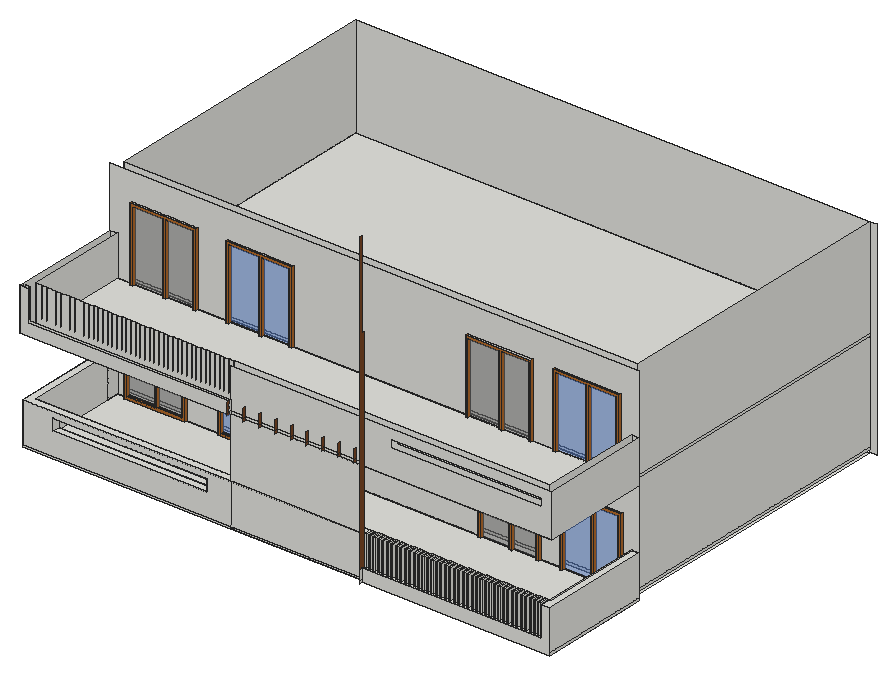
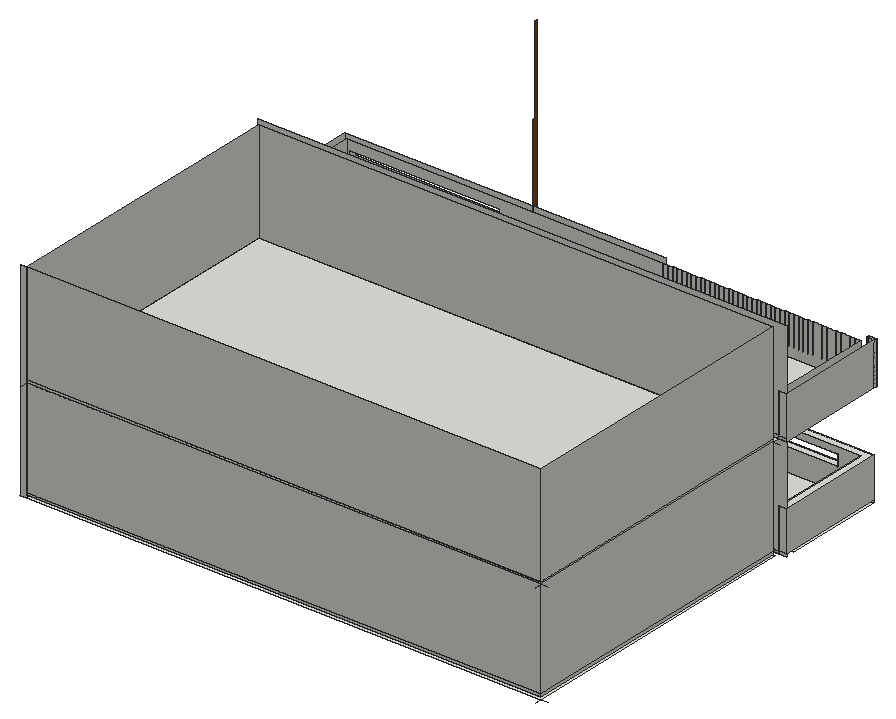
# SketchUp Ruby script. Lengths in inches.
U = 1.inch
M = Sketchup.active_model
def pt(a) = Geom::Point3d.new(a.map { |v| v * U })
def face(e, loops, mat)
  f = e.add_face(loops[0].map { |a| pt(a) })
  loops[1..].each { |l| e.add_face(l.map { |a| pt(a) }).erase! }
  f.material = f.back_material = mat if mat
  f
end
# faces: each face lists its corners as indices into pts; further lists are holes
def faces(e, pts, list, mat = nil) = list.each { |f| face(e, (f[0].is_a?(Array) ? f : [f]).map { |l| l.map { |i| pts[i] } }, mat) }
# xy, xz, yz: faces in a plane at the given z, y or x. An outline is a flat list of corners, or four numbers for a rectangle; further outlines are holes
def ring(l) = l.size == 4 ? [[l[0], l[1]], [l[2], l[1]], [l[2], l[3]], [l[0], l[3]]] : l.each_slice(2).to_a
def flat(e, list, mat, &to3) = list.each { |f| face(e, (f[0].is_a?(Array) ? f : [f]).map { |l| ring(l).map { |u, v| to3.(u, v) } }, mat) }
def xy(e, z, list, mat = nil) = flat(e, list, mat) { |x, y| [x, y, z] }
def xz(e, y, list, mat = nil) = flat(e, list, mat) { |x, z| [x, y, z] }
def yz(e, x, list, mat = nil) = flat(e, list, mat) { |y, z| [x, y, z] }
def lines(e, pts, list) = list.each { |a, b| e.add_line(pt(pts[a]), pt(pts[b])) }
# prism: a flat outline (further loops are holes) pulled along v
def prism(e, loops, v, mat = nil)
  f = face(e, loops, mat); d = Geom::Vector3d.new(v.map { |x| x * U })
  f.pushpull(f.normal.samedirection?(d) ? d.length : -d.length)
end
def box(e, o, s, mat = nil) = prism(e, [[o, [o[0] + s[0], o[1], o[2]], [o[0] + s[0], o[1] + s[1], o[2]], [o[0], o[1] + s[1], o[2]]]], [0, 0, s[2]], mat)
def at(x, y, z, deg = 0) = Geom::Transformation.translation(pt([x, y, z])) * Geom::Transformation.rotation(ORIGIN, Z_AXIS, deg.degrees)
def axes(o, x, y, z) = Geom::Transformation.new([*x, 0, *y, 0, *z, 0, *pt(o).to_a, 1])
def part(name) = M.definitions.add(name)
# library, detail: a bought-in or finely detailed component or shape, given as its bounding box
def library(name, o, s) = part(name).tap { |d| box(d.entities, o, s) }
def detail(e, o, s) = box(e.add_group.entities, o, s)
def put(e, d, t, mat = nil) = e.add_instance(d, t).tap { |i| i.material = mat if mat }
def group(e, t, mat = nil) = e.add_group.tap { |g| g.transformation = t; g.material = mat if mat }.entities
root = M.entities
M.materials.add("[Translucent Glass Blue]").color = [100, 149, 237]
M.materials["[Translucent Glass Blue]"].alpha = 0.5
M.materials.add("[Translucent Glass Gray]").color = [128, 128, 128]
M.materials["[Translucent Glass Gray]"].alpha = 0.5
M.materials.add("[Wood Bamboo]").color = [177, 105, 43]
M.materials.add("[Wood Veneer 01]").color = [120, 70, 37]
xy(root,366,[[9,142.3125,621,490.375]])
xy(root,366.375,[[406.875,3,406.875,6,0,6,0,126.125,630,126.125,630,3],[9,126.125,620.5,136.3125],[620.5,126.125,621,136.3125],[621,126.125,629.5625,136.3125],[629.5625,126.125,630,136.3125]])
xy(root,369,[[9,15,621,15,621,136.3125,610.3125,136.3125,610.3125,133.3125,607.3125,133.3125,607.3125,136.3125,577.78,136.3125,577.78,133.3125,574.3125,133.3125,574.3125,136.3125,541.3125,136.3125,541.3125,133.3125,538.3125,133.3125,538.3125,136.3125,512.74,136.3125,512.74,133.3125,509.74,133.3125,509.74,136.3125,480.64,136.3125,480.64,133.3125,476.74,133.3125,476.74,136.3125,443.74,136.3125,443.74,133.3125,440.74,133.3125,440.74,136.3125,203.05,136.3125,203.05,133.3125,131.05,133.3125,131.05,136.3125,91.27,136.3125,91.27,133.3125,19.27,133.3125,19.27,136.3125,9,136.3125],[19.27,133.3125,91.27,136.3125],[131.05,133.3125,203.05,136.3125],[440.74,133.3125,443.74,136.3125],[476.74,133.3125,480.64,136.3125],
  [509.74,133.3125,512.74,136.3125],[538.3125,133.3125,541.3125,136.3125],[574.3125,133.3125,577.78,136.3125],[607.3125,133.3125,610.3125,136.3125],[9,145.3125,621,490.375]])
xy(root,372,[[134.05,133.3125,167.05,136.3125],[170.54,133.3125,200.05,136.3125]])
xy(root,372,[[22.27,133.3125,55.27,136.3125],[58.04,133.3125,88.27,136.3125]],"[Wood Bamboo]")
xy(root,381.34,[[406.875,3,619.375,3,619.375,15,616.68,15,616.68,6,614.0625,6,614.0625,15,611.37,15,611.37,6,608.75,6,608.75,15,606.06,15,606.06,6,603.4375,6,603.4375,15,600.74,15,600.74,6,598.125,6,598.125,15,595.43,15,595.43,6,592.8125,6,592.8125,15,590.12,15,590.12,6,587.5,6,587.5,15,584.81,15,584.81,6,582.1875,6,582.1875,15,579.49,15,579.49,6,576.875,6,576.875,15,574.18,15,574.18,6,571.5625,6,571.5625,15,568.87,15,568.87,6,566.25,6,566.25,15,563.56,15,563.56,6,560.9375,6,560.9375,15,558.24,15,558.24,6,555.625,6,555.625,15,552.93,15,552.93,6,550.3125,6,550.3125,15,547.62,15,547.62,6,545,6,545,15,542.31,15,542.31,6,539.6875,6,539.6875,15,536.99,15,536.99,6,534.375,6,534.375,15,531.68,15,531.68,6,529.0625,6,529.0625,15,526.37,15,526.37,6,523.75,6,523.75,15,521.06,15,521.06,6,518.4375,6,518.4375,15,515.74,15,515.74,6,513.125,6,513.125,15,510.43,15,510.43,6,507.8125,6,507.8125,15,505.12,15,505.12,6,502.5,6,502.5,15,499.81,15,499.81,6,497.1875,6,497.1875,15,494.49,15,494.49,6,491.875,6,491.875,15,489.18,15,489.18,6,486.5625,6,486.5625,15,483.87,15,483.87,6,481.25,6,481.25,15,478.56,15,478.56,6,475.9375,6,475.9375,15,473.24,15,473.24,6,470.625,6,470.625,15,467.93,15,467.93,6,465.3125,6,465.3125,15,462.62,15,462.62,6,460,6,460,15,457.31,15,457.31,6,454.6875,6,454.6875,15,451.99,15,451.99,6,449.375,6,449.375,15,446.68,15,446.68,6,444.0625,6,444.0625,15,441.37,15,441.37,6,438.75,6,438.75,15,436.06,15,436.06,6,433.4375,6,433.4375,15,430.74,15,430.74,6,428.125,6,428.125,15,425.43,15,425.43,6,422.8125,6,422.8125,15,420.12,15,420.12,6,417.5,6,417.5,15,414.81,15,414.81,6,412.1875,6,412.1875,15,409.49,15,409.49,6,406.875,6]])
xy(root,395.98,[[36.51,6,219.89,15]])
xy(root,410.04,[[36.51,6,219.89,15]])
xy(root,417,[[619.375,3,630,3,630,136.3125,621,136.3125,621,15,619.375,15],[0,6,406.875,6,406.875,15,9,15,9,136.3125,0,136.3125],[406.875,6,409.49,15],[412.1875,6,414.81,15],[417.5,6,420.12,15],
  [422.8125,6,425.43,15],[428.125,6,430.74,15],[433.4375,6,436.06,15],[438.75,6,441.37,15],[444.0625,6,446.68,15],
  [449.375,6,451.99,15],[454.6875,6,457.31,15],[460,6,462.62,15],[465.3125,6,467.93,15],[470.625,6,473.24,15],
  [475.9375,6,478.56,15],[481.25,6,483.87,15],[486.5625,6,489.18,15],[491.875,6,494.49,15],[497.1875,6,499.81,15],
  [502.5,6,505.12,15],[507.8125,6,510.43,15],[513.125,6,515.74,15],[518.4375,6,521.06,15],[523.75,6,526.37,15],
  [529.0625,6,531.68,15],[534.375,6,536.99,15],[539.6875,6,542.31,15],[545,6,547.62,15],[550.3125,6,552.93,15],
  [555.625,6,558.24,15],[560.9375,6,563.56,15],[566.25,6,568.87,15],[571.5625,6,574.18,15],[576.875,6,579.49,15],
  [582.1875,6,584.81,15],[587.5,6,590.12,15],[592.8125,6,595.43,15],[598.125,6,600.74,15],[603.4375,6,606.06,15],
  [608.75,6,611.37,15],[614.0625,6,616.68,15]])
xy(root,450,[[22.27,133.3125,55.27,136.3125],[58.04,133.3125,88.27,136.3125]])
xy(root,450,[[134.05,133.3125,167.05,136.3125],[170.54,133.3125,200.05,136.3125],[443.74,133.3125,476.74,136.3125],[480.64,133.3125,509.74,136.3125],[541.3125,133.3125,574.3125,136.3125],
  [577.78,133.3125,607.3125,136.3125]],"[Wood Bamboo]")
xy(root,453,[[19.27,133.3125,91.27,136.3125],[131.05,133.3125,203.05,136.3125],[440.74,133.3125,512.74,136.3125],[538.3125,133.3125,610.3125,136.3125]],"[Wood Bamboo]")
xy(root,489,[[0,3,248.625,6],[0,6,621,136.3125],[621,6,630,136.3125],[9,136.3125,621,145.3125],[9,145.3125,621,490.375]])
xy(root,492,[[9,145.3125,621,490.375]])
xy(root,492.5625,[[9,15,621,15,621,136.3125,607.86,136.3125,607.86,133.3125,604.86,133.3125,604.86,136.3125,572.23,136.3125,572.23,133.3125,568.86,133.3125,568.86,136.3125,532.86,136.3125,532.86,133.3125,529.86,133.3125,529.86,136.3125,503.86,136.3125,503.86,133.3125,500.86,133.3125,500.86,136.3125,469.18,136.3125,469.18,133.3125,464.86,133.3125,464.86,136.3125,428.86,136.3125,428.86,133.3125,425.86,133.3125,425.86,136.3125,218.85,136.3125,218.85,133.3125,215.85,133.3125,215.85,136.3125,182.97,136.3125,182.97,133.3125,179.85,133.3125,179.85,136.3125,143.85,136.3125,143.85,133.3125,140.85,133.3125,140.85,136.3125,104.31,136.3125,104.31,133.3125,101.31,133.3125,101.31,136.3125,69.34,136.3125,69.34,133.3125,65.31,133.3125,65.31,136.3125,29.31,136.3125,29.31,133.3125,26.31,133.3125,26.31,136.3125,9,136.3125],[26.31,133.3125,29.31,136.3125],[65.31,133.3125,69.34,136.3125],[101.31,133.3125,104.31,136.3125],[140.85,133.3125,143.85,136.3125],
  [179.85,133.3125,182.97,136.3125],[215.85,133.3125,218.85,136.3125],[425.86,133.3125,428.86,136.3125],[464.86,133.3125,469.18,136.3125],[500.86,133.3125,503.86,136.3125],
  [529.86,133.3125,532.86,136.3125],[568.86,133.3125,572.23,136.3125],[604.86,133.3125,607.86,136.3125]])
xz(root,3,[[406.875,366.375,630,366.375,630,417,619.375,417,619.375,381.34,406.875,381.34],[0,489,248.625,489,248.625,503.6,9.45,503.6,9.45,540,0,540]])
xz(root,6,[[248.625,366,406.875,366.375],[0,366.375,248.625,369],[248.625,366.375,406.875,369],[[0,369,248.625,417],[36.51,395.98,219.89,410.04]],[248.625,369,406.875,417],
  [406.875,381.34,409.49,417],[412.1875,381.34,414.81,417],[417.5,381.34,420.12,417],[422.8125,381.34,425.43,417],[428.125,381.34,430.74,417],
  [433.4375,381.34,436.06,417],[438.75,381.34,441.37,417],[444.0625,381.34,446.68,417],[449.375,381.34,451.99,417],[454.6875,381.34,457.31,417],
  [460,381.34,462.62,417],[465.3125,381.34,467.93,417],[470.625,381.34,473.24,417],[475.9375,381.34,478.56,417],[481.25,381.34,483.87,417],
  [486.5625,381.34,489.18,417],[491.875,381.34,494.49,417],[497.1875,381.34,499.81,417],[502.5,381.34,505.12,417],[507.8125,381.34,510.43,417],
  [513.125,381.34,515.74,417],[518.4375,381.34,521.06,417],[523.75,381.34,526.37,417],[529.0625,381.34,531.68,417],[534.375,381.34,536.99,417],
  [539.6875,381.34,542.31,417],[545,381.34,547.62,417],[550.3125,381.34,552.93,417],[555.625,381.34,558.24,417],[560.9375,381.34,563.56,417],
  [566.25,381.34,568.87,417],[571.5625,381.34,574.18,417],[576.875,381.34,579.49,417],[582.1875,381.34,584.81,417],[587.5,381.34,590.12,417],
  [592.8125,381.34,595.43,417],[598.125,381.34,600.74,417],[603.4375,381.34,606.06,417],[608.75,381.34,611.37,417],[614.0625,381.34,616.68,417],
  [248.625,417,406.875,489],[0,489,0,540,0.61,540,0.61,503.6,3.875,503.6,3.875,540,6.17,540,6.17,503.6,9.4375,503.6,9.4375,540,9.45,540,9.45,503.6,248.625,503.6,248.625,489],[248.625,489,406.875,492],[[406.875,489,630,540],[439.02,519.5625,618.46,529]],[248.625,492,406.875,540]])
xz(root,15,[[[9,369,248.625,417],[36.51,395.98,219.89,410.04]],[248.625,369,406.875,417],[406.875,369,406.875,417,409.49,417,409.49,381.34,412.1875,381.34,412.1875,417,414.81,417,414.81,381.34,417.5,381.34,417.5,417,420.12,417,420.12,381.34,422.8125,381.34,422.8125,417,425.43,417,425.43,381.34,428.125,381.34,428.125,417,430.74,417,430.74,381.34,433.4375,381.34,433.4375,417,436.06,417,436.06,381.34,438.75,381.34,438.75,417,441.37,417,441.37,381.34,444.0625,381.34,444.0625,417,446.68,417,446.68,381.34,449.375,381.34,449.375,417,451.99,417,451.99,381.34,454.6875,381.34,454.6875,417,457.31,417,457.31,381.34,460,381.34,460,417,462.62,417,462.62,381.34,465.3125,381.34,465.3125,417,467.93,417,467.93,381.34,470.625,381.34,470.625,417,473.24,417,473.24,381.34,475.9375,381.34,475.9375,417,478.56,417,478.56,381.34,481.25,381.34,481.25,417,483.87,417,483.87,381.34,486.5625,381.34,486.5625,417,489.18,417,489.18,381.34,491.875,381.34,491.875,417,494.49,417,494.49,381.34,497.1875,381.34,497.1875,417,499.81,417,499.81,381.34,502.5,381.34,502.5,417,505.12,417,505.12,381.34,507.8125,381.34,507.8125,417,510.43,417,510.43,381.34,513.125,381.34,513.125,417,515.74,417,515.74,381.34,518.4375,381.34,518.4375,417,521.06,417,521.06,381.34,523.75,381.34,523.75,417,526.37,417,526.37,381.34,529.0625,381.34,529.0625,417,531.68,417,531.68,381.34,534.375,381.34,534.375,417,536.99,417,536.99,381.34,539.6875,381.34,539.6875,417,542.31,417,542.31,381.34,545,381.34,545,417,547.62,417,547.62,381.34,550.3125,381.34,550.3125,417,552.93,417,552.93,381.34,555.625,381.34,555.625,417,558.24,417,558.24,381.34,560.9375,381.34,560.9375,417,563.56,417,563.56,381.34,566.25,381.34,566.25,417,568.87,417,568.87,381.34,571.5625,381.34,571.5625,417,574.18,417,574.18,381.34,576.875,381.34,576.875,417,579.49,417,579.49,381.34,582.1875,381.34,582.1875,417,584.81,417,584.81,381.34,587.5,381.34,587.5,417,590.12,417,590.12,381.34,592.8125,381.34,592.8125,417,595.43,417,595.43,381.34,598.125,381.34,598.125,417,600.74,417,600.74,381.34,603.4375,381.34,603.4375,417,606.06,417,606.06,381.34,608.75,381.34,608.75,417,611.37,417,611.37,381.34,614.0625,381.34,614.0625,417,616.68,417,616.68,381.34,619.375,381.34,619.375,417,621,417,621,369],[[9,492.5625,9,540,9.45,540,9.45,503.6,11.73,503.6,11.73,540,15,540,15,503.6,17.29,503.6,17.29,540,20.5625,540,20.5625,503.6,22.86,503.6,22.86,540,26.125,540,26.125,503.6,28.42,503.6,28.42,540,31.6875,540,31.6875,503.6,33.98,503.6,33.98,540,37.25,540,37.25,503.6,39.54,503.6,39.54,540,42.8125,540,42.8125,503.6,45.11,503.6,45.11,540,48.375,540,48.375,503.6,50.67,503.6,50.67,540,53.9375,540,53.9375,503.6,56.23,503.6,56.23,540,59.5,540,59.5,503.6,61.79,503.6,61.79,540,65.0625,540,65.0625,503.6,67.36,503.6,67.36,540,70.625,540,70.625,503.6,72.92,503.6,72.92,540,76.1875,540,76.1875,503.6,78.48,503.6,78.48,540,81.75,540,81.75,503.6,84.04,503.6,84.04,540,87.3125,540,87.3125,503.6,89.61,503.6,89.61,540,92.875,540,92.875,503.6,95.17,503.6,95.17,540,98.4375,540,98.4375,503.6,100.73,503.6,100.73,540,104,540,104,503.6,106.29,503.6,106.29,540,109.5625,540,109.5625,503.6,111.86,503.6,111.86,540,115.125,540,115.125,503.6,117.42,503.6,117.42,540,120.6875,540,120.6875,503.6,122.98,503.6,122.98,540,126.25,540,126.25,503.6,128.54,503.6,128.54,540,131.8125,540,131.8125,503.6,134.11,503.6,134.11,540,137.375,540,137.375,503.6,139.67,503.6,139.67,540,142.9375,540,142.9375,503.6,145.23,503.6,145.23,540,148.5,540,148.5,503.6,150.79,503.6,150.79,540,154.0625,540,154.0625,503.6,156.36,503.6,156.36,540,159.625,540,159.625,503.6,161.92,503.6,161.92,540,165.1875,540,165.1875,503.6,167.48,503.6,167.48,540,170.75,540,170.75,503.6,173.04,503.6,173.04,540,176.3125,540,176.3125,503.6,178.61,503.6,178.61,540,181.875,540,181.875,503.6,184.17,503.6,184.17,540,187.4375,540,187.4375,503.6,189.73,503.6,189.73,540,193,540,193,503.6,195.29,503.6,195.29,540,198.5625,540,198.5625,503.6,200.86,503.6,200.86,540,204.125,540,204.125,503.6,206.42,503.6,206.42,540,209.6875,540,209.6875,503.6,211.98,503.6,211.98,540,215.25,540,215.25,503.6,217.54,503.6,217.54,540,220.8125,540,220.8125,503.6,223.11,503.6,223.11,540,226.375,540,226.375,503.6,228.67,503.6,228.67,540,231.9375,540,231.9375,503.6,234.23,503.6,234.23,540,237.5,540,237.5,503.6,239.79,503.6,239.79,540,243.0625,540,243.0625,503.6,245.36,503.6,245.36,540,621,540,621,492.5625],[439.02,519.5625,618.46,529]]])
xz(root,133.3125,[[[19.27,369,91.27,453],[22.27,372,55.27,450],[58.04,372,88.27,450]],[[131.05,369,203.05,453],[134.05,372,167.05,450],[170.54,372,200.05,450]],[440.74,369,443.74,369,443.74,450,476.74,450,476.74,369,480.64,369,480.64,450,509.74,450,509.74,369,512.74,369,512.74,453,440.74,453],[538.3125,369,541.3125,369,541.3125,450,574.3125,450,574.3125,369,577.78,369,577.78,450,607.3125,450,607.3125,369,610.3125,369,610.3125,453,538.3125,453],[26.31,492.5625,29.31,492.5625,29.31,576.5625,65.31,576.5625,65.31,492.5625,69.34,492.5625,69.34,576.5625,101.31,576.5625,101.31,492.5625,104.31,492.5625,104.31,579.5625,26.31,579.5625],
  [140.85,492.5625,143.85,492.5625,143.85,576.5625,179.85,576.5625,179.85,492.5625,182.97,492.5625,182.97,576.5625,215.85,576.5625,215.85,492.5625,218.85,492.5625,218.85,579.5625,140.85,579.5625],[425.86,492.5625,428.86,492.5625,428.86,576.5625,464.86,576.5625,464.86,492.5625,469.18,492.5625,469.18,576.5625,500.86,576.5625,500.86,492.5625,503.86,492.5625,503.86,579.5625,425.86,579.5625],[529.86,492.5625,532.86,492.5625,532.86,576.5625,568.86,576.5625,568.86,492.5625,572.23,492.5625,572.23,576.5625,604.86,576.5625,604.86,492.5625,607.86,492.5625,607.86,579.5625,529.86,579.5625]],"[Wood Bamboo]")
xz(root,136.3125,[[0,366,9,369],[9,366.375,620.5,369],[620.5,366.375,621,369],[621,366.375,629.5625,369],[629.5625,366.375,630,369],
  [0,369,9,417],[9,369,19.27,369,19.27,453,91.27,453,91.27,369,131.05,369,131.05,453,203.05,453,203.05,369,440.74,369,440.74,453,512.74,453,512.74,369,538.3125,369,538.3125,453,610.3125,453,610.3125,369,621,369,621,417,630,417,630,489,0,489,0,417,9,417],[[19.27,369,91.27,453],[22.27,372,55.27,450],[58.04,372,88.27,450]],[[131.05,369,203.05,453],[134.05,372,167.05,450],[170.54,372,200.05,450]],[440.74,369,440.74,453,512.74,453,512.74,369,509.74,369,509.74,450,480.64,450,480.64,369,476.74,369,476.74,450,443.74,450,443.74,369],
  [538.3125,369,538.3125,453,610.3125,453,610.3125,369,607.3125,369,607.3125,450,577.78,450,577.78,369,574.3125,369,574.3125,450,541.3125,450,541.3125,369],[621,369,629.5625,417],[629.5625,369,630,417],[0,489,9,492],[9,489,620.5,489,620.5,492.5625,607.86,492.5625,607.86,489.5625,529.86,489.5625,529.86,492.5625,503.86,492.5625,503.86,489.5625,425.86,489.5625,425.86,492.5625,218.85,492.5625,218.85,489.5625,140.85,489.5625,140.85,492.5625,104.31,492.5625,104.31,489.5625,26.31,489.5625,26.31,492.5625,9,492.5625],
  [620.5,489,621,492.5625],[621,489,629.5625,492],[629.5625,489,630,492],[26.31,489.5625,104.31,492.5625],[140.85,489.5625,218.85,492.5625],
  [425.86,489.5625,503.86,492.5625],[529.86,489.5625,607.86,492.5625],[0,492,9,540],[621,492,629.5625,540],[629.5625,492,630,540],
  [9,492.5625,26.31,492.5625,26.31,579.5625,104.31,579.5625,104.31,492.5625,140.85,492.5625,140.85,579.5625,218.85,579.5625,218.85,492.5625,425.86,492.5625,425.86,579.5625,503.86,579.5625,503.86,492.5625,529.86,492.5625,529.86,579.5625,607.86,579.5625,607.86,492.5625,621,492.5625,621,540,630,540,630,612,0,612,0,540,9,540],[26.31,492.5625,26.31,579.5625,104.31,579.5625,104.31,492.5625,101.31,492.5625,101.31,576.5625,69.34,576.5625,69.34,492.5625,65.31,492.5625,65.31,576.5625,29.31,576.5625,29.31,492.5625],[140.85,492.5625,140.85,579.5625,218.85,579.5625,218.85,492.5625,215.85,492.5625,215.85,576.5625,182.97,576.5625,182.97,492.5625,179.85,492.5625,179.85,576.5625,143.85,576.5625,143.85,492.5625],[425.86,492.5625,425.86,579.5625,503.86,579.5625,503.86,492.5625,500.86,492.5625,500.86,576.5625,469.18,576.5625,469.18,492.5625,464.86,492.5625,464.86,576.5625,428.86,576.5625,428.86,492.5625],[529.86,492.5625,529.86,579.5625,607.86,579.5625,607.86,492.5625,604.86,492.5625,604.86,576.5625,572.23,576.5625,572.23,492.5625,568.86,492.5625,568.86,576.5625,532.86,576.5625,532.86,492.5625]])
xz(root,136.3125,[[541.3125,369,574.3125,450],[577.78,369,607.3125,450],[134.05,372,167.05,450],[170.54,372,200.05,450],[143.85,492.5625,179.85,576.5625],
  [182.97,492.5625,215.85,576.5625],[532.86,492.5625,568.86,576.5625],[572.23,492.5625,604.86,576.5625]],"[Translucent Glass Blue]")
xz(root,136.3125,[[443.74,369,476.74,450],[480.64,369,509.74,450],[22.27,372,55.27,450],[58.04,372,88.27,450],[29.31,492.5625,65.31,576.5625],
  [69.34,492.5625,101.31,576.5625],[428.86,492.5625,464.86,576.5625],[469.18,492.5625,500.86,576.5625]],"[Translucent Glass Gray]")
xz(root,145.3125,[[9,369,621,372],[9,372,621,489],[9,489,621,492],[9,492,621,612]])
xz(root,490.375,[[620.75,366,628.8125,366,628.8125,612,621,612,621,369,620.75,369],[9,369,620.75,372],[620.75,369,621,372],[9,372,620.75,489],[620.75,372,621,489],
  [9,489,620.75,492],[620.75,489,621,492],[9,492,620.75,612],[620.75,492,621,612]])
yz(root,0,[[6,369,136.3125,417],[3,489,6,540],[6,489,136.3125,540]])
yz(root,9,[[126.125,366,136.3125,366.375],[121.57,366.375,136.3125,369],[15,369,121.57,417],[121.57,369,136.3125,417],[145.3125,369,490.375,372],
  [145.3125,372,490.375,489],[145.3125,489,490.375,492],[145.3125,492,490.375,612],[15,492.5625,136.3125,540]])
yz(root,19.27,[[133.3125,369,136.3125,453]],"[Wood Bamboo]")
yz(root,22.27,[[133.3125,372,136.3125,450]],"[Wood Bamboo]")
yz(root,26.31,[[133.3125,492.5625,136.3125,579.5625]],"[Wood Bamboo]")
yz(root,29.31,[[133.3125,492.5625,136.3125,576.5625]],"[Wood Bamboo]")
yz(root,36.51,[[6,395.98,15,410.04]])
yz(root,55.27,[[133.3125,372,136.3125,450]],"[Wood Bamboo]")
yz(root,58.04,[[133.3125,372,136.3125,450]],"[Wood Bamboo]")
yz(root,65.31,[[133.3125,492.5625,136.3125,576.5625]],"[Wood Bamboo]")
yz(root,69.34,[[133.3125,492.5625,136.3125,576.5625]],"[Wood Bamboo]")
yz(root,88.27,[[133.3125,372,136.3125,450]],"[Wood Bamboo]")
yz(root,91.27,[[133.3125,369,136.3125,453]],"[Wood Bamboo]")
yz(root,101.31,[[133.3125,492.5625,136.3125,576.5625]],"[Wood Bamboo]")
yz(root,104.31,[[133.3125,492.5625,136.3125,579.5625]],"[Wood Bamboo]")
yz(root,131.05,[[133.3125,369,136.3125,453]],"[Wood Bamboo]")
yz(root,134.05,[[133.3125,372,136.3125,450]],"[Wood Bamboo]")
yz(root,140.85,[[133.3125,492.5625,136.3125,579.5625]],"[Wood Bamboo]")
yz(root,143.85,[[133.3125,492.5625,136.3125,576.5625]],"[Wood Bamboo]")
yz(root,167.05,[[133.3125,372,136.3125,450]],"[Wood Bamboo]")
yz(root,170.54,[[133.3125,372,136.3125,450]],"[Wood Bamboo]")
yz(root,179.85,[[133.3125,492.5625,136.3125,576.5625]],"[Wood Bamboo]")
yz(root,182.97,[[133.3125,492.5625,136.3125,576.5625]],"[Wood Bamboo]")
yz(root,200.05,[[133.3125,372,136.3125,450]],"[Wood Bamboo]")
yz(root,203.05,[[133.3125,369,136.3125,453]],"[Wood Bamboo]")
yz(root,215.85,[[133.3125,492.5625,136.3125,576.5625]],"[Wood Bamboo]")
yz(root,218.85,[[133.3125,492.5625,136.3125,579.5625]],"[Wood Bamboo]")
yz(root,219.89,[[6,395.98,15,410.04]])
yz(root,248.625,[[3,489,6,492],[3,492,6,503.6]])
yz(root,248.625,[[0,489,3,492],[0,492,3,503.6]],"[Wood Veneer 01]")
yz(root,267.4375,[[0,489.375,3,492.375],[0,492.375,3,503.98]],"[Wood Veneer 01]")
yz(root,286.25,[[0,489.75,3,492.75],[0,492.75,3,504.35]],"[Wood Veneer 01]")
yz(root,305.06,[[0,490.125,3,493.125],[0,493.125,3,504.73]],"[Wood Veneer 01]")
yz(root,323.87,[[0,490.5,3,493.5],[0,493.5,3,505.1]],"[Wood Veneer 01]")
yz(root,342.68,[[0,490.875,3,493.875],[0,493.875,3,505.48]],"[Wood Veneer 01]")
yz(root,361.49,[[0,491.25,3,494.25],[0,494.25,3,505.85]],"[Wood Veneer 01]")
yz(root,380.31,[[0,491.625,3,494.625],[0,494.625,3,506.23]],"[Wood Veneer 01]")
yz(root,399.12,[[0,492,3,495],[0,495,3,506.6]],"[Wood Veneer 01]")
yz(root,406.875,[[0,366.375,3,369],[3,366.375,6,369],[0,369,3,381.34],[3,369,6,381.34]])
yz(root,406.875,[[0,381.34,6,381.34,6,632.0625,3,632.0625,3,735.4375,0,735.4375]],"[Wood Veneer 01]")
yz(root,409.49,[[6,381.34,15,417]])
yz(root,412.1875,[[6,381.34,15,417]])
yz(root,414.81,[[6,381.34,15,417]])
yz(root,417.5,[[6,381.34,15,417]])
yz(root,420.12,[[6,381.34,15,417]])
yz(root,422.8125,[[6,381.34,15,417]])
yz(root,425.43,[[6,381.34,15,417]])
yz(root,425.86,[[133.3125,492.5625,136.3125,579.5625]],"[Wood Bamboo]")
yz(root,428.125,[[6,381.34,15,417]])
yz(root,428.86,[[133.3125,492.5625,136.3125,576.5625]],"[Wood Bamboo]")
yz(root,430.74,[[6,381.34,15,417]])
yz(root,433.4375,[[6,381.34,15,417]])
yz(root,436.06,[[6,381.34,15,417]])
yz(root,438.75,[[6,381.34,15,417]])
yz(root,440.74,[[133.3125,369,136.3125,453]],"[Wood Bamboo]")
yz(root,441.37,[[6,381.34,15,417]])
yz(root,443.74,[[133.3125,369,136.3125,450]],"[Wood Bamboo]")
yz(root,444.0625,[[6,381.34,15,417]])
yz(root,446.68,[[6,381.34,15,417]])
yz(root,449.375,[[6,381.34,15,417]])
yz(root,451.99,[[6,381.34,15,417]])
yz(root,454.6875,[[6,381.34,15,417]])
yz(root,457.31,[[6,381.34,15,417]])
yz(root,460,[[6,381.34,15,417]])
yz(root,462.62,[[6,381.34,15,417]])
yz(root,464.86,[[133.3125,492.5625,136.3125,576.5625]],"[Wood Bamboo]")
yz(root,465.3125,[[6,381.34,15,417]])
yz(root,467.93,[[6,381.34,15,417]])
yz(root,469.18,[[133.3125,492.5625,136.3125,576.5625]],"[Wood Bamboo]")
yz(root,470.625,[[6,381.34,15,417]])
yz(root,473.24,[[6,381.34,15,417]])
yz(root,475.9375,[[6,381.34,15,417]])
yz(root,476.74,[[133.3125,369,136.3125,450]],"[Wood Bamboo]")
yz(root,478.56,[[6,381.34,15,417]])
yz(root,480.64,[[133.3125,369,136.3125,450]],"[Wood Bamboo]")
yz(root,481.25,[[6,381.34,15,417]])
yz(root,483.87,[[6,381.34,15,417]])
yz(root,486.5625,[[6,381.34,15,417]])
yz(root,489.18,[[6,381.34,15,417]])
yz(root,491.875,[[6,381.34,15,417]])
yz(root,494.49,[[6,381.34,15,417]])
yz(root,497.1875,[[6,381.34,15,417]])
yz(root,499.81,[[6,381.34,15,417]])
yz(root,500.86,[[133.3125,492.5625,136.3125,576.5625]],"[Wood Bamboo]")
yz(root,502.5,[[6,381.34,15,417]])
yz(root,503.86,[[133.3125,492.5625,136.3125,579.5625]],"[Wood Bamboo]")
yz(root,505.12,[[6,381.34,15,417]])
yz(root,507.8125,[[6,381.34,15,417]])
yz(root,509.74,[[133.3125,369,136.3125,450]],"[Wood Bamboo]")
yz(root,510.43,[[6,381.34,15,417]])
yz(root,512.74,[[133.3125,369,136.3125,453]],"[Wood Bamboo]")
yz(root,513.125,[[6,381.34,15,417]])
yz(root,515.74,[[6,381.34,15,417]])
yz(root,518.4375,[[6,381.34,15,417]])
yz(root,521.06,[[6,381.34,15,417]])
yz(root,523.75,[[6,381.34,15,417]])
yz(root,526.37,[[6,381.34,15,417]])
yz(root,529.0625,[[6,381.34,15,417]])
yz(root,529.86,[[133.3125,492.5625,136.3125,579.5625]],"[Wood Bamboo]")
yz(root,531.68,[[6,381.34,15,417]])
yz(root,532.86,[[133.3125,492.5625,136.3125,576.5625]],"[Wood Bamboo]")
yz(root,534.375,[[6,381.34,15,417]])
yz(root,536.99,[[6,381.34,15,417]])
yz(root,538.3125,[[133.3125,369,136.3125,453]],"[Wood Bamboo]")
yz(root,539.6875,[[6,381.34,15,417]])
yz(root,541.3125,[[133.3125,369,136.3125,450]],"[Wood Bamboo]")
yz(root,542.31,[[6,381.34,15,417]])
yz(root,545,[[6,381.34,15,417]])
yz(root,547.62,[[6,381.34,15,417]])
yz(root,550.3125,[[6,381.34,15,417]])
yz(root,552.93,[[6,381.34,15,417]])
yz(root,555.625,[[6,381.34,15,417]])
yz(root,558.24,[[6,381.34,15,417]])
yz(root,560.9375,[[6,381.34,15,417]])
yz(root,563.56,[[6,381.34,15,417]])
yz(root,566.25,[[6,381.34,15,417]])
yz(root,568.86,[[133.3125,492.5625,136.3125,576.5625]],"[Wood Bamboo]")
yz(root,568.87,[[6,381.34,15,417]])
yz(root,571.5625,[[6,381.34,15,417]])
yz(root,572.23,[[133.3125,492.5625,136.3125,576.5625]],"[Wood Bamboo]")
yz(root,574.18,[[6,381.34,15,417]])
yz(root,574.3125,[[133.3125,369,136.3125,450]],"[Wood Bamboo]")
yz(root,576.875,[[6,381.34,15,417]])
yz(root,577.78,[[133.3125,369,136.3125,450]],"[Wood Bamboo]")
yz(root,579.49,[[6,381.34,15,417]])
yz(root,582.1875,[[6,381.34,15,417]])
yz(root,584.81,[[6,381.34,15,417]])
yz(root,587.5,[[6,381.34,15,417]])
yz(root,590.12,[[6,381.34,15,417]])
yz(root,592.8125,[[6,381.34,15,417]])
yz(root,595.43,[[6,381.34,15,417]])
yz(root,598.125,[[6,381.34,15,417]])
yz(root,600.74,[[6,381.34,15,417]])
yz(root,603.4375,[[6,381.34,15,417]])
yz(root,604.86,[[133.3125,492.5625,136.3125,576.5625]],"[Wood Bamboo]")
yz(root,606.06,[[6,381.34,15,417]])
yz(root,607.3125,[[133.3125,369,136.3125,450]],"[Wood Bamboo]")
yz(root,607.86,[[133.3125,492.5625,136.3125,579.5625]],"[Wood Bamboo]")
yz(root,608.75,[[6,381.34,15,417]])
yz(root,610.3125,[[133.3125,369,136.3125,453]],"[Wood Bamboo]")
yz(root,611.37,[[6,381.34,15,417]])
yz(root,614.0625,[[6,381.34,15,417]])
yz(root,616.68,[[6,381.34,15,417]])
yz(root,619.375,[[3,381.34,15,417]])
yz(root,621,[[15,369,127.3125,417],[127.3125,369,136.3125,417],[145.3125,369,490.375,372],[145.3125,372,490.375,489],[145.3125,489,490.375,492],
  [145.3125,492,490.375,612],[15,492.5625,136.3125,540]])
yz(root,630,[[3,366.375,136.3125,369],[3,369,136.3125,417],[6,489,136.3125,540]])
p = [[621,136.3125,366],[621,142.3125,366],[9,490.375,366],[9,499.375,366],[0,490.375,366],[9,490.375,489],
  [9,499.375,489],[621,490.375,489],[621,499.375,489],[0,490.375,489],[9,145.3125,489],[0,145.3125,489],
  [621,136.3125,366.375],[628.8125,490.375,366],[630,490.375,366],[621,127.3125,369],[620.5,127.3125,369]]
lines(root,p,[[0,1],[2,3],[2,4],[5,6],[7,8],[5,9],[10,11],[12,0],[13,14],[15,16]])
